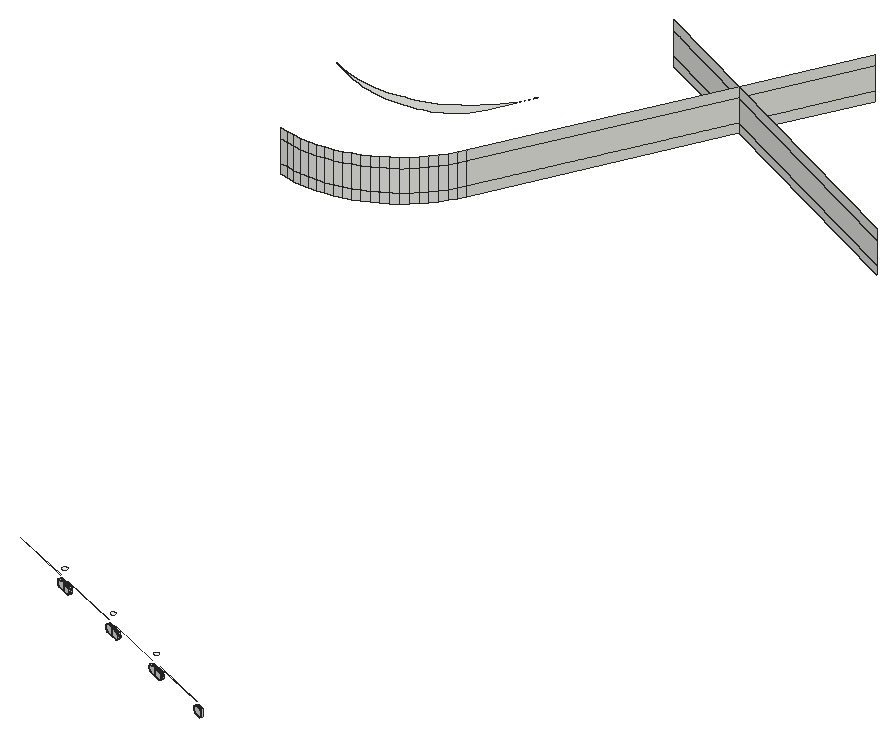
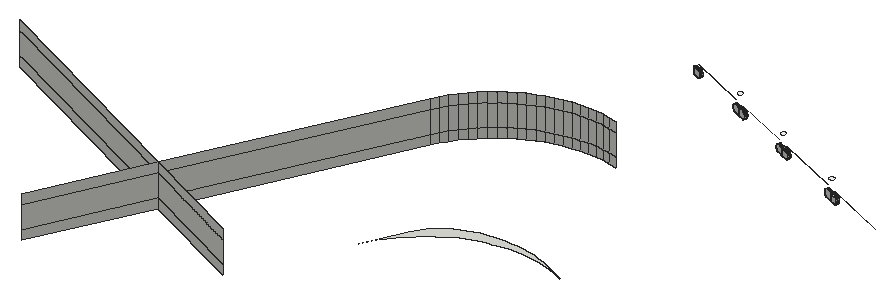
# SketchUp Ruby script. Lengths in inches.
U = 1.inch
M = Sketchup.active_model
def pt(a) = Geom::Point3d.new(a.map { |v| v * U })
def face(e, loops, mat)
  f = e.add_face(loops[0].map { |a| pt(a) })
  loops[1..].each { |l| e.add_face(l.map { |a| pt(a) }).erase! }
  f.material = f.back_material = mat if mat
  f
end
# faces: each face lists its corners as indices into pts; further lists are holes
def faces(e, pts, list, mat = nil) = list.each { |f| face(e, (f[0].is_a?(Array) ? f : [f]).map { |l| l.map { |i| pts[i] } }, mat) }
# xy, xz, yz: faces in a plane at the given z, y or x. An outline is a flat list of corners, or four numbers for a rectangle; further outlines are holes
def ring(l) = l.size == 4 ? [[l[0], l[1]], [l[2], l[1]], [l[2], l[3]], [l[0], l[3]]] : l.each_slice(2).to_a
def flat(e, list, mat, &to3) = list.each { |f| face(e, (f[0].is_a?(Array) ? f : [f]).map { |l| ring(l).map { |u, v| to3.(u, v) } }, mat) }
def xy(e, z, list, mat = nil) = flat(e, list, mat) { |x, y| [x, y, z] }
def xz(e, y, list, mat = nil) = flat(e, list, mat) { |x, z| [x, y, z] }
def yz(e, x, list, mat = nil) = flat(e, list, mat) { |y, z| [x, y, z] }
def lines(e, pts, list) = list.each { |a, b| e.add_line(pt(pts[a]), pt(pts[b])) }
# prism: a flat outline (further loops are holes) pulled along v
def prism(e, loops, v, mat = nil)
  f = face(e, loops, mat); d = Geom::Vector3d.new(v.map { |x| x * U })
  f.pushpull(f.normal.samedirection?(d) ? d.length : -d.length)
end
def box(e, o, s, mat = nil) = prism(e, [[o, [o[0] + s[0], o[1], o[2]], [o[0] + s[0], o[1] + s[1], o[2]], [o[0], o[1] + s[1], o[2]]]], [0, 0, s[2]], mat)
def at(x, y, z, deg = 0) = Geom::Transformation.translation(pt([x, y, z])) * Geom::Transformation.rotation(ORIGIN, Z_AXIS, deg.degrees)
def axes(o, x, y, z) = Geom::Transformation.new([*x, 0, *y, 0, *z, 0, *pt(o).to_a, 1])
def part(name) = M.definitions.add(name)
# library, detail: a bought-in or finely detailed component or shape, given as its bounding box
def library(name, o, s) = part(name).tap { |d| box(d.entities, o, s) }
def detail(e, o, s) = box(e.add_group.entities, o, s)
def put(e, d, t, mat = nil) = e.add_instance(d, t).tap { |i| i.material = mat if mat }
def group(e, t, mat = nil) = e.add_group.tap { |g| g.transformation = t; g.material = mat if mat }.entities
root = M.entities
M.materials.add("Glass_Safety_01").color = [204, 235, 244]
M.materials["Glass_Safety_01"].alpha = 0.1
M.materials.add("[Color_000]").color = [255, 255, 255]
xy(root,351.28,[[786.9,558.15,785.1,558.9375,785.21,559.1875,785.36,559.12,787.01,558.4],[787.09,558.58,785.44,559.3,785.29,559.37,785.4,559.62,787.2,558.84],[767.73,566.5,765.93,567.29,766.04,567.54,767.84,566.75],[767.92,566.93,766.12,567.72,766.23,567.97,768.03,567.19],[765.93,567.29,764.12,568.07,764.23,568.32,764.39,568.25,766.04,567.54],
  [766.12,567.72,764.47,568.43,764.3125,568.5,764.42,568.76,766.23,567.97],[747.39,575.36,745.58,576.15,745.69,576.4,747.5,575.61],[747.57,575.79,745.77,576.58,745.88,576.83,747.68,576.05],[745.58,576.15,743.78,576.93,743.89,577.19,744.03,577.12,745.69,576.4],[745.77,576.58,744.11,577.3,743.96,577.37,744.07,577.62,745.88,576.83],
  [724.68,585.25,722.875,586.04,722.99,586.29,724.79,585.5],[724.87,585.68,723.0625,586.47,723.17,586.72,724.98,585.94],[722.875,586.04,721.07,586.82,721.18,587.07,721.33,587.01,722.99,586.29],[723.0625,586.47,721.4,587.19,721.26,587.25,721.37,587.51,723.17,586.72]])
xy(root,351.36,[[787.01,558.4,785.57,559.03,785.65,559.21,787.09,558.58],[767.48,566.91,766.04,567.54,766.12,567.72,767.56,567.09],[766.04,567.54,764.59,568.17,764.67,568.35,766.12,567.72],[747.13,575.77,745.69,576.4,745.77,576.58,747.21,575.95],[745.69,576.4,744.25,577.03,744.33,577.21,745.77,576.58],
  [724.43,585.66,722.99,586.29,723.0625,586.47,724.51,585.84],[722.99,586.29,721.54,586.92,721.62,587.1,723.0625,586.47]],"Glass_Safety_01")
xy(root,353.33,[[787.01,558.4,787.09,558.58,785.65,559.21,785.57,559.03],[767.48,566.91,767.56,567.09,766.12,567.72,766.04,567.54],[766.04,567.54,766.12,567.72,764.67,568.35,764.59,568.17],[747.13,575.77,747.21,575.95,745.77,576.58,745.69,576.4],[745.69,576.4,745.77,576.58,744.33,577.21,744.25,577.03],
  [724.43,585.66,724.51,585.84,723.0625,586.47,722.99,586.29],[722.99,586.29,723.0625,586.47,721.62,587.1,721.54,586.92]],"Glass_Safety_01")
xy(root,353.41,[[786.9,558.15,787.01,558.4,785.36,559.12,785.21,559.1875,785.1,558.9375],[787.09,558.58,787.2,558.84,785.4,559.62,785.29,559.37,785.44,559.3],[767.73,566.5,767.84,566.75,766.04,567.54,765.93,567.29],[767.92,566.93,768.03,567.19,766.23,567.97,766.12,567.72],[765.93,567.29,766.04,567.54,764.39,568.25,764.23,568.32,764.12,568.07],
  [766.12,567.72,766.23,567.97,764.42,568.76,764.3125,568.5,764.47,568.43],[747.39,575.36,747.5,575.61,745.69,576.4,745.58,576.15],[747.57,575.79,747.68,576.05,745.88,576.83,745.77,576.58],[745.58,576.15,745.69,576.4,744.03,577.12,743.89,577.19,743.78,576.93],[745.77,576.58,745.88,576.83,744.07,577.62,743.96,577.37,744.11,577.3],
  [724.68,585.25,724.79,585.5,722.99,586.29,722.875,586.04],[724.87,585.68,724.98,585.94,723.17,586.72,723.0625,586.47],[722.875,586.04,722.99,586.29,721.33,587.01,721.18,587.07,721.07,586.82],[723.0625,586.47,723.17,586.72,721.37,587.51,721.26,587.25,721.4,587.19]])
xy(root,354.51,[[785.36,559.12,785.44,559.3,767.84,566.75],[785.44,559.3,767.92,566.93,767.84,566.75],[764.39,568.25,764.47,568.43,747.5,575.61],[764.47,568.43,747.57,575.79,747.5,575.61],[744.03,577.12,744.11,577.3,724.79,585.5],
  [744.11,577.3,724.87,585.68,724.79,585.5],[721.33,587.01,721.4,587.19,702.27,595.31],[721.4,587.19,702.35,595.49,702.27,595.31]],"Glass_Safety_01")
xy(root,357.27,[[766.12,567,766.28,567.03,766.43,567.11,766.55,567.22,766.64,567.35,766.69,567.51,766.7,567.67,766.67,567.83,766.6,567.98,766.49,568.1,766.35,568.19,766.2,568.25,766.03,568.26,765.87,568.22,765.72,568.15,765.6,568.04,765.51,567.9,765.46,567.75,765.45,567.58,765.48,567.42,765.55,567.28,765.66,567.15,765.8,567.0625,765.96,567.01],[745.78,575.86,745.9375,575.89,746.08,575.97,746.21,576.08,746.3,576.21,746.35,576.37,746.36,576.53,746.33,576.7,746.25,576.84,746.14,576.97,746.01,577.06,745.85,577.11,745.68,577.12,745.52,577.08,745.375,577.01,745.25,576.9,745.16,576.76,745.11,576.61,745.1,576.44,745.13,576.28,745.21,576.14,745.32,576.01,745.45,575.92,745.61,575.87],[723.07,585.75,723.23,585.78,723.38,585.86,723.5,585.97,723.59,586.1,723.64,586.26,723.65,586.42,723.62,586.58,723.55,586.73,723.4375,586.85,723.3,586.95,723.14,587,722.98,587.01,722.82,586.97,722.67,586.9,722.55,586.79,722.46,586.65,722.41,586.5,722.4,586.33,722.43,586.17,722.5,586.03,722.61,585.9,722.75,585.8125,722.91,585.76]],"[Color_000]")
xy(root,412.84,[[703.25,736.11,701.35,736.17,699.43,736.32,697.49,736.59,695.54,736.95,693.59,737.42,691.66,737.98,689.74,738.64,687.85,739.4,685.99,740.25,681.68,742.34,683.83,741.38,686.04,740.57,688.3,739.9,690.59,739.375,692.92,739.01,695.27,738.79,697.62,738.73,699.98,738.82,702.32,739.06,704.64,739.46,706.02,739.79,706.96,739.93,708.44,740.24,709.88,740.65,711.25,741.13,712.5625,741.7,713.8,742.36,714.96,743.09,716.04,743.89,716.26,744.08,717.58,744.92,719.49,746.3,721.3,747.81,723.01,749.43,724.61,751.16,726.1,752.99,727.46,754.91,728.6875,756.92,729.79,759,723.97,747.02,723.26,745.72,722.43,744.47,721.5,743.3,720.45,742.2,719.29,741.1875,718.04,740.25,716.69,739.4,715.25,738.65,713.73,737.98,712.14,737.42,710.47,736.95,708.74,736.59,706.96,736.32,705.125,736.17]])
p = [[786.9,558.15,353.41],[785.1,558.9375,353.41],[784.85,559.05,353.37],[784.61,559.15,353.27],[784.41,559.24,353.1],[784.25,559.3,352.88],
  [784.16,559.35,352.62],[784.125,559.36,352.35],[784.16,559.35,352.07],[784.25,559.3,351.81],[784.41,559.24,351.59],[784.61,559.15,351.43],
  [784.85,559.05,351.32],[785.1,558.9375,351.28],[786.9,558.15,351.28],[787.01,558.4,351.28],[785.36,559.12,351.28],[785.36,559.12,353.41],
  [787.01,558.4,353.41],[787.01,558.4,353.33],[785.57,559.03,353.33],[785.57,559.03,351.36],[787.01,558.4,351.36],[787.09,558.58,353.41],
  [785.44,559.3,353.41],[785.44,559.3,351.28],[787.09,558.58,351.28],[787.09,558.58,351.36],[785.65,559.21,351.36],[785.65,559.21,353.33],
  [787.09,558.58,353.33],[787.2,558.84,351.28],[787.2,558.84,353.41],[785.4,559.62,353.41],[785.4,559.62,351.28],[785.14,559.73,351.32],
  [784.91,559.83,351.43],[784.71,559.92,351.59],[784.55,559.99,351.81],[784.46,560.03,352.07],[784.42,560.05,352.35],[784.46,560.03,352.62],
  [784.55,559.99,352.88],[784.71,559.92,353.1],[784.91,559.83,353.27],[785.14,559.73,353.37],[784.96,559.3,351.32],[785.21,559.1875,351.28],
  [784.72,559.4,351.43],[785.21,559.1875,353.41],[784.52,559.49,351.59],[784.36,559.56,351.81],[784.27,559.6,352.07],[784.23,559.61,352.35],
  [784.27,559.6,352.62],[784.36,559.56,352.88],[784.52,559.49,353.1],[784.72,559.4,353.27],[784.96,559.3,353.37],[785.29,559.37,351.28],
  [785.29,559.37,353.41],[785.03,559.48,353.37],[784.8,559.58,353.27],[784.6,559.67,353.1],[784.44,559.74,352.88],[784.35,559.78,352.62],
  [784.3125,559.79,352.35],[784.35,559.78,352.07],[784.44,559.74,351.81],[784.6,559.67,351.59],[784.8,559.58,351.43],[785.03,559.48,351.32],
  [767.73,566.5,353.41],[765.93,567.29,353.41],[765.93,567.29,351.28],[767.73,566.5,351.28],[767.98,566.39,351.32],[768.22,566.29,351.43],
  [768.42,566.2,351.59],[768.58,566.13,351.81],[768.67,566.09,352.07],[768.71,566.07,352.35],[768.67,566.09,352.62],[768.58,566.13,352.88],
  [768.42,566.2,353.1],[768.22,566.29,353.27],[767.98,566.39,353.37],[767.84,566.75,353.41],[767.84,566.75,351.28],[768.09,566.64,351.32],
  [768.33,566.54,351.43],[768.53,566.45,351.59],[768.6875,566.38,351.81],[768.78,566.34,352.07],[768.82,566.33,352.35],[768.78,566.34,352.62],
  [768.6875,566.38,352.88],[768.53,566.45,353.1],[768.33,566.54,353.27],[768.09,566.64,353.37],[767.92,566.93,351.28],[767.92,566.93,353.41],
  [768.17,566.82,353.37],[768.41,566.72,353.27],[768.61,566.63,353.1],[768.76,566.56,352.88],[768.86,566.52,352.62],[768.89,566.51,352.35],
  [768.86,566.52,352.07],[768.76,566.56,351.81],[768.61,566.63,351.59],[768.41,566.72,351.43],[768.17,566.82,351.32],[768.28,567.08,351.32],
  [768.52,566.97,351.43],[766.04,567.54,353.41],[766.04,567.54,351.28],[766.04,567.54,351.36],[767.48,566.91,351.36],[767.48,566.91,353.33],
  [766.04,567.54,353.33],[766.23,567.97,353.41],[768.03,567.19,353.41],[768.28,567.08,353.37],[768.52,566.97,353.27],[768.72,566.88,353.1],
  [768.875,566.82,352.88],[768.97,566.78,352.62],[769,566.76,352.35],[768.97,566.78,352.07],[768.875,566.82,351.81],[768.72,566.88,351.59],
  [768.03,567.19,351.28],[766.23,567.97,351.28],[766.12,567.72,351.28],[766.12,567.72,353.41],[766.12,567.72,353.33],[767.56,567.09,353.33],
  [767.56,567.09,351.36],[766.12,567.72,351.36],[764.12,568.07,353.41],[763.87,568.18,353.37],[763.63,568.28,353.27],[763.43,568.37,353.1],
  [763.28,568.4375,352.88],[763.18,568.48,352.62],[763.15,568.5,352.35],[763.18,568.48,352.07],[763.28,568.4375,351.81],[763.43,568.37,351.59],
  [763.63,568.28,351.43],[763.87,568.18,351.32],[764.12,568.07,351.28],[764.39,568.25,351.28],[764.39,568.25,353.41],[764.59,568.17,353.33],
  [764.59,568.17,351.36],[764.47,568.43,353.41],[764.47,568.43,351.28],[764.67,568.35,351.36],[764.67,568.35,353.33],[764.42,568.76,353.41],
  [764.42,568.76,351.28],[764.17,568.87,351.32],[763.93,568.97,351.43],[763.73,569.06,351.59],[763.58,569.125,351.81],[763.48,569.17,352.07],
  [763.45,569.18,352.35],[763.48,569.17,352.62],[763.58,569.125,352.88],[763.73,569.06,353.1],[763.93,568.97,353.27],[764.17,568.87,353.37],
  [763.98,568.43,351.32],[764.23,568.32,351.28],[763.74,568.54,351.43],[764.23,568.32,353.41],[763.54,568.625,351.59],[763.39,568.69,351.81],
  [763.29,568.73,352.07],[763.26,568.75,352.35],[763.29,568.73,352.62],[763.39,568.69,352.88],[763.54,568.625,353.1],[763.74,568.54,353.27],
  [763.98,568.43,353.37],[764.3125,568.5,351.28],[764.3125,568.5,353.41],[764.06,568.61,353.37],[763.82,568.72,353.27],[763.62,568.8,353.1],
  [763.47,568.87,352.88],[763.37,568.91,352.62],[763.34,568.93,352.35],[763.37,568.91,352.07],[763.47,568.87,351.81],[763.62,568.8,351.59],
  [763.82,568.72,351.43],[764.06,568.61,351.32],[747.39,575.36,353.41],[745.58,576.15,353.41],[745.58,576.15,351.28],[747.39,575.36,351.28],
  [747.64,575.25,351.32],[747.87,575.15,351.43],[748.07,575.0625,351.59],[748.23,574.99,351.81],[748.33,574.95,352.07],[748.36,574.9375,352.35],
  [748.33,574.95,352.62],[748.23,574.99,352.88],[748.07,575.0625,353.1],[747.87,575.15,353.27],[747.64,575.25,353.37],[747.75,575.5,351.32],
  [747.98,575.4,351.43],[747.5,575.61,353.41],[747.5,575.61,351.28],[748.18,575.3125,351.59],[748.34,575.25,351.81],[748.4375,575.2,352.07],
  [748.47,575.1875,352.35],[748.4375,575.2,352.62],[748.34,575.25,352.88],[748.18,575.3125,353.1],[747.98,575.4,353.27],[747.75,575.5,353.37],
  [747.57,575.79,351.28],[747.57,575.79,353.41],[747.83,575.68,353.37],[748.0625,575.58,353.27],[748.26,575.49,353.1],[748.42,575.43,352.88],
  [748.52,575.38,352.62],[748.55,575.37,352.35],[748.52,575.38,352.07],[748.42,575.43,351.81],[748.26,575.49,351.59],[748.0625,575.58,351.43],
  [747.83,575.68,351.32],[745.69,576.4,353.41],[745.69,576.4,351.28],[745.69,576.4,351.36],[747.13,575.77,351.36],[747.13,575.77,353.33],
  [745.69,576.4,353.33],[745.88,576.83,353.41],[747.68,576.05,353.41],[747.9375,575.9375,353.37],[748.17,575.83,353.27],[748.375,575.75,353.1],
  [748.53,575.68,352.88],[748.625,575.64,352.62],[748.66,575.62,352.35],[748.625,575.64,352.07],[748.53,575.68,351.81],[748.375,575.75,351.59],
  [748.17,575.83,351.43],[747.9375,575.9375,351.32],[747.68,576.05,351.28],[745.88,576.83,351.28],[745.77,576.58,351.28],[745.77,576.58,353.41],
  [745.77,576.58,353.33],[747.21,575.95,353.33],[747.21,575.95,351.36],[745.77,576.58,351.36],[743.78,576.93,353.41],[743.52,577.04,353.37],
  [743.29,577.15,353.27],[743.09,577.23,353.1],[742.93,577.3,352.88],[742.83,577.34,352.62],[742.8,577.36,352.35],[742.83,577.34,352.07],
  [742.93,577.3,351.81],[743.09,577.23,351.59],[743.29,577.15,351.43],[743.52,577.04,351.32],[743.78,576.93,351.28],[744.03,577.12,351.28],
  [744.03,577.12,353.41],[744.25,577.03,353.33],[744.25,577.03,351.36],[744.11,577.3,353.41],[744.11,577.3,351.28],[744.33,577.21,351.36],
  [744.33,577.21,353.33],[744.07,577.62,353.41],[744.07,577.62,351.28],[743.82,577.73,351.32],[743.59,577.83,351.43],[743.39,577.92,351.59],
  [743.23,577.99,351.81],[743.13,578.03,352.07],[743.1,578.04,352.35],[743.13,578.03,352.62],[743.23,577.99,352.88],[743.39,577.92,353.1],
  [743.59,577.83,353.27],[743.82,577.73,353.37],[743.63,577.3,351.32],[743.89,577.19,351.28],[743.4,577.4,351.43],[743.89,577.19,353.41],
  [743.2,577.49,351.59],[743.04,577.55,351.81],[742.94,577.6,352.07],[742.91,577.61,352.35],[742.94,577.6,352.62],[743.04,577.55,352.88],
  [743.2,577.49,353.1],[743.4,577.4,353.27],[743.63,577.3,353.37],[743.96,577.37,351.28],[743.96,577.37,353.41],[743.71,577.48,353.37],
  [743.48,577.58,353.27],[743.28,577.67,353.1],[743.12,577.73,352.88],[743.02,577.78,352.62],[742.99,577.79,352.35],[743.02,577.78,352.07],
  [743.12,577.73,351.81],[743.28,577.67,351.59],[743.48,577.58,351.43],[743.71,577.48,351.32],[724.68,585.25,353.41],[722.875,586.04,353.41],
  [722.875,586.04,351.28],[724.68,585.25,351.28],[724.93,585.14,351.32],[725.17,585.04,351.43],[725.37,584.95,351.59],[725.52,584.88,351.81],
  [725.62,584.84,352.07],[725.65,584.83,352.35],[725.62,584.84,352.62],[725.52,584.88,352.88],[725.37,584.95,353.1],[725.17,585.04,353.27],
  [724.93,585.14,353.37],[725.04,585.39,351.32],[725.28,585.29,351.43],[724.79,585.5,351.28],[724.79,585.5,353.41],[725.48,585.2,351.59],
  [725.63,585.13,351.81],[725.73,585.09,352.07],[725.76,585.08,352.35],[725.73,585.09,352.62],[725.63,585.13,352.88],[725.48,585.2,353.1],
  [725.28,585.29,353.27],[725.04,585.39,353.37],[724.87,585.68,351.28],[724.87,585.68,353.41],[725.12,585.57,353.37],[725.36,585.47,353.27],
  [725.56,585.38,353.1],[725.71,585.32,352.88],[725.81,585.27,352.62],[725.84,585.26,352.35],[725.81,585.27,352.07],[725.71,585.32,351.81],
  [725.56,585.38,351.59],[725.36,585.47,351.43],[725.12,585.57,351.32],[722.99,586.29,353.41],[722.99,586.29,351.28],[722.99,586.29,351.36],
  [724.43,585.66,351.36],[724.43,585.66,353.33],[722.99,586.29,353.33],[723.17,586.72,353.41],[724.98,585.94,353.41],[725.23,585.83,353.37],
  [725.47,585.72,353.27],[725.67,585.64,353.1],[725.82,585.57,352.88],[725.92,585.53,352.62],[725.95,585.51,352.35],[725.92,585.53,352.07],
  [725.82,585.57,351.81],[725.67,585.64,351.59],[725.47,585.72,351.43],[725.23,585.83,351.32],[724.98,585.94,351.28],[723.17,586.72,351.28],
  [723.0625,586.47,351.28],[723.0625,586.47,353.41],[723.0625,586.47,353.33],[724.51,585.84,353.33],[724.51,585.84,351.36],[723.0625,586.47,351.36],
  [721.07,586.82,353.41],[720.82,586.93,353.37],[720.58,587.03,353.27],[720.38,587.12,353.1],[720.23,587.1875,352.88],[720.13,587.23,352.62],
  [720.1,587.25,352.35],[720.13,587.23,352.07],[720.23,587.1875,351.81],[720.38,587.12,351.59],[720.58,587.03,351.43],[720.82,586.93,351.32],
  [721.07,586.82,351.28],[721.33,587.01,351.28],[721.33,587.01,353.41],[721.54,586.92,353.33],[721.54,586.92,351.36],[721.4,587.19,353.41],
  [721.4,587.19,351.28],[721.62,587.1,351.36],[721.62,587.1,353.33],[721.37,587.51,353.41],[721.37,587.51,351.28],[721.12,587.62,351.32],
  [720.88,587.72,351.43],[720.68,587.81,351.59],[720.53,587.875,351.81],[720.43,587.92,352.07],[720.39,587.93,352.35],[720.43,587.92,352.62],
  [720.53,587.875,352.88],[720.68,587.81,353.1],[720.88,587.72,353.27],[721.12,587.62,353.37],[720.93,587.18,351.32],[721.18,587.07,351.28],
  [720.69,587.29,351.43],[721.18,587.07,353.41],[720.49,587.375,351.59],[720.34,587.44,351.81],[720.24,587.48,352.07],[720.21,587.5,352.35],
  [720.24,587.48,352.62],[720.34,587.44,352.88],[720.49,587.375,353.1],[720.69,587.29,353.27],[720.93,587.18,353.37],[721.26,587.25,351.28],
  [721.26,587.25,353.41],[721.01,587.36,353.37],[720.77,587.47,353.27],[720.57,587.55,353.1],[720.42,587.62,352.88],[720.32,587.66,352.62],
  [720.28,587.68,352.35],[720.32,587.66,352.07],[720.42,587.62,351.81],[720.57,587.55,351.59],[720.77,587.47,351.43],[721.01,587.36,351.32],
  [711.93,690.68,415.76],[711.93,690.68,412.84],[714.28,690.62,412.84],[714.28,690.62,415.76],[716.63,690.71,412.84],[716.63,690.71,415.76],
  [709.58,690.9,415.76],[709.58,690.9,412.84],[718.98,690.96,412.84],[718.98,690.96,415.76],[707.25,691.27,415.76],[707.25,691.27,412.84],
  [721.3,691.35,412.84],[721.3,691.35,415.76],[704.96,691.79,415.76],[704.96,691.79,412.84],[723.59,691.9,412.84],[723.59,691.9,415.76],
  [725.84,692.6,412.84],[725.84,692.6,415.76],[728.04,693.44,412.84],[728.04,693.44,415.76],[730.18,694.43,412.84],[730.18,694.43,415.76],
  [732.25,695.55,412.84],[732.25,695.55,415.76],[734.24,696.81,412.84],[734.24,696.81,415.76],[736.15,698.19,412.84],[736.15,698.19,415.76],
  [737.96,699.7,412.84],[737.96,699.7,415.76],[739.67,701.32,412.84],[739.67,701.32,415.76],[741.27,703.05,412.84],[741.27,703.05,415.76],
  [742.75,704.88,412.84],[742.75,704.88,415.76],[744.12,706.8,412.84],[744.12,706.8,415.76],[745.35,708.81,412.84],[745.35,708.81,415.76],
  [746.44,710.89,412.84],[746.44,710.89,415.76],[777.88,775.64,412.84],[793.61,808.02,412.84],[793.61,808.02,415.76],[777.88,775.64,415.76],
  [745.5,791.36,415.76],[745.5,791.36,412.84],[846.87,742.14,412.84],[846.87,742.14,415.76],[714.28,690.62,422.51],[711.93,690.68,422.51],
  [716.63,690.71,422.51],[709.58,690.9,422.51],[718.98,690.96,422.51],[707.25,691.27,422.51],[721.3,691.35,422.51],[704.96,691.79,422.51],
  [723.59,691.9,422.51],[725.84,692.6,422.51],[728.04,693.44,422.51],[730.18,694.43,422.51],[732.25,695.55,422.51],[734.24,696.81,422.51],
  [736.15,698.19,422.51],[737.96,699.7,422.51],[739.67,701.32,422.51],[741.27,703.05,422.51],[742.75,704.88,422.51],[744.12,706.8,422.51],
  [745.35,708.81,422.51],[746.44,710.89,422.51],[793.61,808.02,422.51],[777.88,775.64,422.51],[846.87,742.14,422.51],[745.5,791.36,422.51],
  [714.28,690.62,425.53],[711.93,690.68,425.53],[716.63,690.71,425.53],[709.58,690.9,425.53],[718.98,690.96,425.53],[707.25,691.27,425.53],
  [721.3,691.35,425.53],[704.96,691.79,425.53],[723.59,691.9,425.53],[725.84,692.6,425.53],[728.04,693.44,425.53],[730.18,694.43,425.53],
  [732.25,695.55,425.53],[734.24,696.81,425.53],[736.15,698.19,425.53],[737.96,699.7,425.53],[739.67,701.32,425.53],[741.27,703.05,425.53],
  [742.75,704.88,425.53],[744.12,706.8,425.53],[745.35,708.81,425.53],[746.44,710.89,425.53],[793.61,808.02,425.53],[777.88,775.64,425.53],
  [846.87,742.14,425.53],[745.5,791.36,425.53]]
faces(root,p,[[0,1,2,3,4,5,6,7,8,9,10,11,12,13,14],[15,16,17,18,19,20,21,22],[23,24,25,26,27,28,29,30],[27,26,31,32,23,30],[33,32,31,34,35,36,37,38,39,40,41,42,43,44,45],[46,47,13,12],[48,46,12,11],[49,17,16,47,46,48,50,51,52,53,54,55,56,57,58],
  [59,25,24,60,61,62,63,64,65,66,67,68,69,70,71],[59,71,35,34],[71,70,36,35],[72,73,74,75,76,77,78,79,80,81,82,83,84,85,86],[89,90,77,76],[88,89,76,75],[111,112,113,114],[115,87,88,116,117,118,119,120],
  [121,122,123,124,125,126,127,128,129,130,131,114,113,132,133],[112,100,132,113],[134,100,101,135,136,137,138,139],[73,140,141,142,143,144,145,146,147,148,149,150,151,152,74],[116,117,120,115,73,74],[116,153,154,115,120,155,156,117],[135,157,158,134,139,159,160,136],[139,134,133,121,135,136],
  [161,121,133,162,163,164,165,166,167,168,169,170,171,172,173],[174,175,152,151],[176,174,151,150],[177,154,153,175,174,176,178,179,180,181,182,183,184,185,186],[187,158,157,188,189,190,191,192,193,194,195,196,197,198,199],[187,199,163,162],[199,198,164,163],[200,201,202,203,204,205,206,207,208,209,210,211,212,213,214],
  [215,216,205,204],[218,215,204,203],[241,217,218,242,243,244,245,246],[247,248,249,250,251,252,253,254,255,256,257,258,259,260,261],[239,240,259,258],[240,228,260,259],[262,228,229,263,264,265,266,267],[201,268,269,270,271,272,273,274,275,276,277,278,279,280,202],
  [242,243,246,241,201,202],[242,281,282,241,246,283,284,243],[263,285,286,262,267,287,288,264],[267,262,261,247,263,264],[289,247,261,290,291,292,293,294,295,296,297,298,299,300,301],[302,303,280,279],[304,302,279,278],[305,282,281,303,302,304,306,307,308,309,310,311,312,313,314],
  [315,286,285,316,317,318,319,320,321,322,323,324,325,326,327],[315,327,291,290],[327,326,292,291],[328,329,330,331,332,333,334,335,336,337,338,339,340,341,342],[343,344,333,332],[345,343,332,331],[369,346,345,370,371,372,373,374],[375,376,377,378,379,380,381,382,383,384,385,386,387,388,389],
  [367,368,387,386],[368,356,388,387],[390,356,357,391,392,393,394,395],[329,396,397,398,399,400,401,402,403,404,405,406,407,408,330],[370,371,374,369,329,330],[370,409,410,369,374,411,412,371],[391,413,414,390,395,415,416,392],[395,390,389,375,391,392],
  [417,375,389,418,419,420,421,422,423,424,425,426,427,428,429],[430,431,408,407],[432,430,407,406],[433,410,409,431,430,432,434,435,436,437,438,439,440,441,442],[443,414,413,444,445,446,447,448,449,450,451,452,453,454,455],[443,455,419,418],[455,454,420,419],[50,48,11,10],
  [70,69,37,36],[90,91,78,77],[110,111,114,131],[178,176,150,149],[198,197,165,164],[216,219,206,205],[238,239,258,257],[306,304,278,277],
  [326,325,293,292],[344,347,334,333],[366,367,386,385],[434,432,406,405],[454,453,421,420],[51,50,10,9],[69,68,38,37],[91,92,79,78],
  [109,110,131,130],[179,178,149,148],[197,196,166,165],[219,220,207,206],[237,238,257,256],[307,306,277,276],[325,324,294,293],[347,348,335,334],
  [365,366,385,384],[435,434,405,404],[453,452,422,421],[52,51,9,8],[68,67,39,38],[92,93,80,79],[108,109,130,129],[180,179,148,147],
  [196,195,167,166],[220,221,208,207],[236,237,256,255],[308,307,276,275],[324,323,295,294],[348,349,336,335],[364,365,384,383],[436,435,404,403],
  [452,451,423,422],[53,52,8,7],[67,66,40,39],[93,94,81,80],[107,108,129,128],[181,180,147,146],[195,194,168,167],[221,222,209,208],
  [235,236,255,254],[309,308,275,274],[323,322,296,295],[349,350,337,336],[363,364,383,382],[437,436,403,402],[451,450,424,423],[54,53,7,6],
  [66,65,41,40],[94,95,82,81],[106,107,128,127],[182,181,146,145],[194,193,169,168],[222,223,210,209],[234,235,254,253],[310,309,274,273],
  [322,321,297,296],[350,351,338,337],[362,363,382,381],[438,437,402,401],[450,449,425,424],[55,54,6,5],[65,64,42,41],[95,96,83,82],
  [105,106,127,126],[183,182,145,144],[193,192,170,169],[223,224,211,210],[233,234,253,252],[311,310,273,272],[321,320,298,297],[351,352,339,338],
  [361,362,381,380],[439,438,401,400],[449,448,426,425],[56,55,5,4],[64,63,43,42],[96,97,84,83],[104,105,126,125],[184,183,144,143],
  [192,191,171,170],[224,225,212,211],[232,233,252,251],[312,311,272,271],[320,319,299,298],[352,353,340,339],[360,361,380,379],[440,439,400,399],
  [448,447,427,426],[57,56,4,3],[63,62,44,43],[97,98,85,84],[103,104,125,124],[185,184,143,142],[191,190,172,171],[225,226,213,212],
  [231,232,251,250],[313,312,271,270],[319,318,300,299],[353,354,341,340],[359,360,379,378],[441,440,399,398],[447,446,428,427],[58,57,3,2],
  [62,61,45,44],[98,99,86,85],[102,103,124,123],[186,185,142,141],[190,189,173,172],[226,227,214,213],[230,231,250,249],[314,313,270,269],
  [318,317,301,300],[354,355,342,341],[358,359,378,377],[442,441,398,397],[446,445,429,428],[49,58,2,1],[61,60,33,45],[99,87,72,86],
  [101,102,123,122],[177,186,141,140],[189,188,161,173],[227,217,200,214],[229,230,249,248],[305,314,269,268],[317,316,289,301],[355,346,328,342],
  [357,358,377,376],[433,442,397,396],[445,444,417,429],[456,457,458,459],[459,458,460,461],[462,463,457,456],[461,460,464,465],[466,467,463,462],
  [465,464,468,469],[470,471,467,466],[469,468,472,473],[473,472,474,475],[475,474,476,477],[477,476,478,479],[479,478,480,481],[481,480,482,483],
  [483,482,484,485],[485,484,486,487],[487,486,488,489],[489,488,490,491],[491,490,492,493],[493,492,494,495],[495,494,496,497],[497,496,498,499],
  [498,500,501,502,503,499],[503,504,505,500,506,507],[456,459,508,509],[459,461,510,508],[462,456,509,511],[461,465,512,510],[466,462,511,513],[465,469,514,512],
  [470,466,513,515],[469,473,516,514],[473,475,517,516],[475,477,518,517],[477,479,519,518],[479,481,520,519],[481,483,521,520],[483,485,522,521],
  [485,487,523,522],[487,489,524,523],[489,491,525,524],[491,493,526,525],[493,495,527,526],[495,497,528,527],[497,499,529,528],[499,503,502,530,531,529],
  [504,503,507,532,531,533],[509,508,534,535],[508,510,536,534],[511,509,535,537],[510,512,538,536],[513,511,537,539],[512,514,540,538],[515,513,539,541],
  [514,516,542,540],[516,517,543,542],[517,518,544,543],[518,519,545,544],[519,520,546,545],[520,521,547,546],[521,522,548,547],[522,523,549,548],
  [523,524,550,549],[524,525,551,550],[525,526,552,551],[526,527,553,552],[527,528,554,553],[528,529,555,554],[529,531,530,556,557,555],[533,531,532,558,557,559]])
faces(root,p,[[87,88,89,90,91,92,93,94,95,96,97,98,99],[100,101,102,103,104,105,106,107,108,109,110,111,112],[217,218,215,216,219,220,221,222,223,224,225,226,227],[228,229,230,231,232,233,234,235,236,237,238,239,240],[346,345,343,344,347,348,349,350,351,352,353,354,355],[356,357,358,359,360,361,362,363,364,365,366,367,368],[20,19,22,21],[30,19,22,27],
  [30,29,28,27],[29,28,21,20],[120,119,118,117],[119,118,138,137],[137,136,139,138],[155,120,117,156],[136,120,117,139],[136,160,159,139],
  [160,159,156,155],[246,245,244,243],[245,244,266,265],[265,264,267,266],[283,246,243,284],[264,246,243,267],[264,288,287,267],[288,287,284,283],
  [374,373,372,371],[373,372,394,393],[393,392,395,394],[411,374,371,412],[392,374,371,395],[392,416,415,395],[416,415,412,411]],"Glass_Safety_01")
